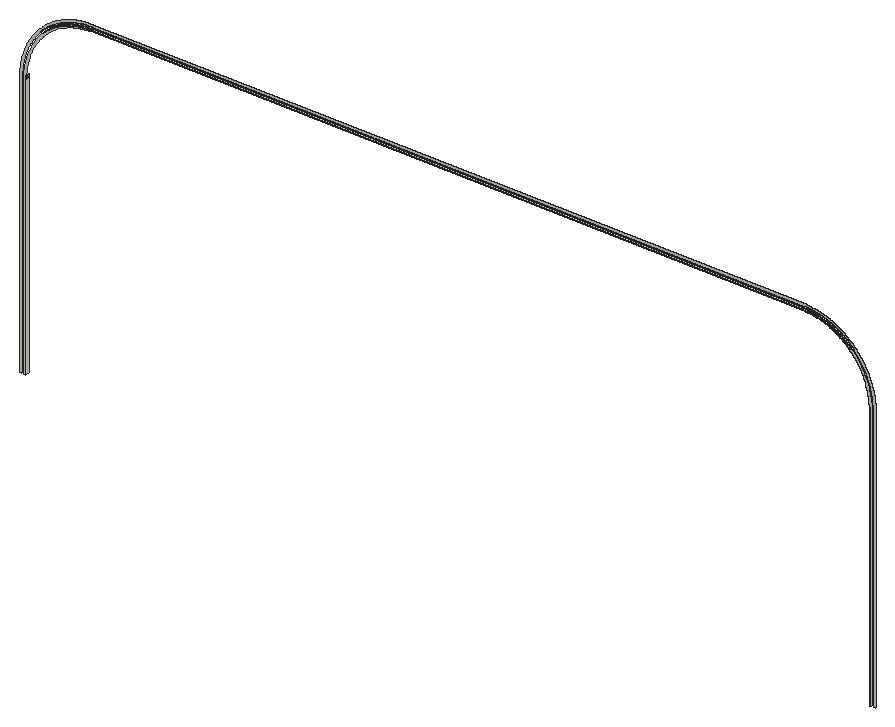
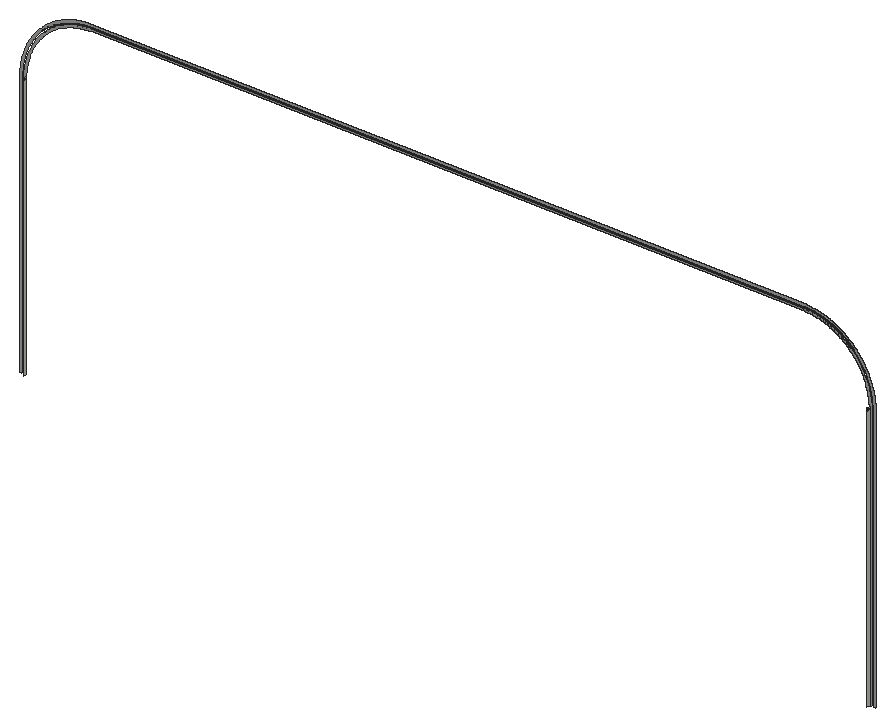
# SketchUp Ruby script. Lengths in inches.
U = 1.inch
M = Sketchup.active_model
def pt(a) = Geom::Point3d.new(a.map { |v| v * U })
def face(e, loops, mat)
  f = e.add_face(loops[0].map { |a| pt(a) })
  loops[1..].each { |l| e.add_face(l.map { |a| pt(a) }).erase! }
  f.material = f.back_material = mat if mat
  f
end
# faces: each face lists its corners as indices into pts; further lists are holes
def faces(e, pts, list, mat = nil) = list.each { |f| face(e, (f[0].is_a?(Array) ? f : [f]).map { |l| l.map { |i| pts[i] } }, mat) }
# xy, xz, yz: faces in a plane at the given z, y or x. An outline is a flat list of corners, or four numbers for a rectangle; further outlines are holes
def ring(l) = l.size == 4 ? [[l[0], l[1]], [l[2], l[1]], [l[2], l[3]], [l[0], l[3]]] : l.each_slice(2).to_a
def flat(e, list, mat, &to3) = list.each { |f| face(e, (f[0].is_a?(Array) ? f : [f]).map { |l| ring(l).map { |u, v| to3.(u, v) } }, mat) }
def xy(e, z, list, mat = nil) = flat(e, list, mat) { |x, y| [x, y, z] }
def xz(e, y, list, mat = nil) = flat(e, list, mat) { |x, z| [x, y, z] }
def yz(e, x, list, mat = nil) = flat(e, list, mat) { |y, z| [x, y, z] }
def lines(e, pts, list) = list.each { |a, b| e.add_line(pt(pts[a]), pt(pts[b])) }
# prism: a flat outline (further loops are holes) pulled along v
def prism(e, loops, v, mat = nil)
  f = face(e, loops, mat); d = Geom::Vector3d.new(v.map { |x| x * U })
  f.pushpull(f.normal.samedirection?(d) ? d.length : -d.length)
end
def box(e, o, s, mat = nil) = prism(e, [[o, [o[0] + s[0], o[1], o[2]], [o[0] + s[0], o[1] + s[1], o[2]], [o[0], o[1] + s[1], o[2]]]], [0, 0, s[2]], mat)
def at(x, y, z, deg = 0) = Geom::Transformation.translation(pt([x, y, z])) * Geom::Transformation.rotation(ORIGIN, Z_AXIS, deg.degrees)
def axes(o, x, y, z) = Geom::Transformation.new([*x, 0, *y, 0, *z, 0, *pt(o).to_a, 1])
def part(name) = M.definitions.add(name)
# library, detail: a bought-in or finely detailed component or shape, given as its bounding box
def library(name, o, s) = part(name).tap { |d| box(d.entities, o, s) }
def detail(e, o, s) = box(e.add_group.entities, o, s)
def put(e, d, t, mat = nil) = e.add_instance(d, t).tap { |i| i.material = mat if mat }
def group(e, t, mat = nil) = e.add_group.tap { |g| g.transformation = t; g.material = mat if mat }.entities
root = M.entities
M.materials.add("[Stone Vein Gray]").color = [206, 202, 201]
xy(root,52.84,[[183.43,83.25,183.57,83.5],[297.43,83.25,297.57,83.5]])
xy(root,52.85,[[183.72,83.25,183.86,83.5],[183.86,83.25,184,83.5],[184,83.25,297,83.5],[297,83.25,297.14,83.5],[297.14,83.25,297.28,83.5]])
xy(root,53.15,[[183.71,83.25,183.85,83.5],[183.85,83.25,184,83.5],[184,83.25,297,83.5],[297,83.25,297.15,83.5],[297.15,83.25,297.29,83.5]])
xz(root,83.5,[[172.5,0,172.5,42.3,172.52,42.6,172.52,42.75,172.54,42.9,172.55,43.05,172.5625,43.2,172.58,43.35,172.64,43.8,172.67,43.95,172.69,44.1,172.72,44.24,172.78,44.54,172.82,44.68,172.85,44.83,172.89,44.98,172.93,45.12,172.97,45.27,173.02,45.41,173.0625,45.55,173.11,45.7,173.26,46.12,173.32,46.26,173.43,46.54,173.49,46.68,173.56,46.81,173.62,46.95,173.6875,47.09,173.75,47.22,173.82,47.35,173.89,47.49,173.97,47.62,174.04,47.75,174.12,47.88,174.19,48.01,174.27,48.14,174.36,48.26,174.4375,48.39,174.52,48.51,174.61,48.64,174.79,48.88,174.875,49,174.97,49.12,175.0625,49.24,175.16,49.35,175.26,49.47,175.35,49.58,175.45,49.7,175.56,49.81,175.66,49.92,176.08,50.34,176.19,50.44,176.3,50.55,176.42,50.65,176.53,50.74,176.65,50.84,176.76,50.9375,176.88,51.03,177,51.125,177.12,51.21,177.36,51.39,177.49,51.48,177.61,51.5625,177.74,51.64,177.86,51.73,177.99,51.81,178.12,51.88,178.25,51.96,178.38,52.03,178.51,52.11,178.65,52.18,178.78,52.25,178.91,52.3125,179.05,52.38,179.19,52.44,179.32,52.51,179.46,52.57,179.74,52.68,179.88,52.74,180.3,52.89,180.45,52.9375,180.59,52.98,180.73,53.03,180.88,53.07,181.02,53.11,181.17,53.15,181.32,53.18,181.46,53.22,181.76,53.28,181.9,53.31,182.05,53.33,182.2,53.36,182.65,53.42,182.8,53.4375,182.95,53.45,183.1,53.46,183.25,53.48,183.4,53.48,183.7,53.5,297.3,53.5,297.6,53.48,297.75,53.48,297.9,53.46,298.05,53.45,298.2,53.4375,298.35,53.42,298.8,53.36,298.95,53.33,299.1,53.31,299.24,53.28,299.54,53.22,299.68,53.18,299.83,53.15,299.98,53.11,300.12,53.07,300.27,53.03,300.41,52.98,300.55,52.9375,300.7,52.89,301.12,52.74,301.26,52.68,301.54,52.57,301.68,52.51,301.81,52.44,301.95,52.38,302.09,52.3125,302.22,52.25,302.35,52.18,302.49,52.11,302.62,52.03,302.75,51.96,302.88,51.88,303.01,51.81,303.14,51.73,303.26,51.64,303.39,51.5625,303.51,51.48,303.64,51.39,303.88,51.21,304,51.125,304.12,51.03,304.24,50.9375,304.35,50.84,304.47,50.74,304.58,50.65,304.7,50.55,304.81,50.44,304.92,50.34,305.34,49.92,305.44,49.81,305.55,49.7,305.65,49.58,305.74,49.47,305.84,49.35,305.9375,49.24,306.03,49.12,306.125,49,306.21,48.88,306.39,48.64,306.48,48.51,306.5625,48.39,306.64,48.26,306.73,48.14,306.81,48.01,306.88,47.88,306.96,47.75,307.03,47.62,307.11,47.49,307.18,47.35,307.25,47.22,307.3125,47.09,307.38,46.95,307.44,46.81,307.51,46.68,307.57,46.54,307.68,46.26,307.74,46.12,307.89,45.7,307.9375,45.55,307.98,45.41,308.03,45.27,308.07,45.12,308.11,44.98,308.15,44.83,308.18,44.68,308.22,44.54,308.28,44.24,308.31,44.1,308.33,43.95,308.36,43.8,308.42,43.35,308.4375,43.2,308.45,43.05,308.46,42.9,308.48,42.75,308.48,42.6,308.5,42.3,308.5,0,308.15,0,308.15,42.29,308.14,42.4375,308.13,42.58,308.125,42.73,308.12,42.875,308.1,43.02,308.09,43.17,308.07,43.3125,308.05,43.46,308.01,43.74,307.99,43.89,307.96,44.03,307.9375,44.18,307.91,44.32,307.84,44.6,307.81,44.74,307.77,44.89,307.65,45.31,307.6,45.45,307.56,45.58,307.41,46,307.36,46.13,307.3,46.27,307.24,46.4,307.1875,46.54,307,46.93,306.93,47.0625,306.87,47.19,306.66,47.58,306.58,47.7,306.51,47.83,306.27,48.19,306.1875,48.32,306.11,48.44,306.02,48.55,305.93,48.67,305.85,48.79,305.76,48.9,305.67,49.02,305.57,49.13,305.48,49.24,305.38,49.35,305.29,49.46,305.1875,49.57,305.09,49.68,304.99,49.78,304.88,49.88,304.78,49.99,304.68,50.09,304.57,50.1875,304.46,50.29,304.35,50.38,304.24,50.48,304.13,50.57,304.02,50.67,303.9,50.76,303.79,50.85,303.67,50.93,303.55,51.02,303.44,51.11,303.32,51.1875,303.19,51.27,302.83,51.51,302.7,51.58,302.58,51.66,302.19,51.87,302.0625,51.93,301.93,52,301.54,52.1875,301.4,52.24,301.27,52.3,301.13,52.36,301,52.41,300.58,52.56,300.45,52.6,300.31,52.65,299.89,52.77,299.74,52.81,299.6,52.84,299.32,52.91,299.18,52.9375,299.03,52.96,298.89,52.99,298.74,53.01,298.46,53.05,298.3125,53.07,298.17,53.09,298.02,53.1,297.875,53.12,297.73,53.125,297.58,53.13,297.4375,53.14,297.29,53.15,183.71,53.15,183.5625,53.14,183.42,53.13,183.27,53.125,183.125,53.12,182.98,53.1,182.83,53.09,182.6875,53.07,182.54,53.05,182.26,53.01,182.11,52.99,181.97,52.96,181.82,52.9375,181.68,52.91,181.4,52.84,181.26,52.81,181.11,52.77,180.69,52.65,180.55,52.6,180.42,52.56,180,52.41,179.87,52.36,179.73,52.3,179.6,52.24,179.46,52.1875,179.07,52,178.9375,51.93,178.81,51.87,178.42,51.66,178.3,51.58,178.17,51.51,177.81,51.27,177.68,51.1875,177.56,51.11,177.45,51.02,177.33,50.93,177.21,50.85,177.1,50.76,176.98,50.67,176.87,50.57,176.76,50.48,176.65,50.38,176.54,50.29,176.43,50.1875,176.32,50.09,176.22,49.99,176.12,49.88,176.01,49.78,175.91,49.68,175.8125,49.57,175.71,49.46,175.62,49.35,175.52,49.24,175.43,49.13,175.33,49.02,175.24,48.9,175.15,48.79,175.07,48.67,174.98,48.55,174.89,48.44,174.8125,48.32,174.73,48.19,174.49,47.83,174.42,47.7,174.34,47.57,174.27,47.45,174.13,47.19,174.07,47.0625,174,46.93,173.8125,46.54,173.76,46.4,173.7,46.27,173.64,46.13,173.59,46,173.44,45.58,173.4,45.45,173.35,45.31,173.23,44.89,173.19,44.74,173.16,44.6,173.09,44.32,173.0625,44.18,173.04,44.03,173.01,43.89,172.99,43.74,172.95,43.46,172.93,43.3125,172.91,43.17,172.9,43.02,172.88,42.875,172.875,42.73,172.87,42.58,172.86,42.4375,172.85,42.29,172.85,0],[173.15,0,173.15,42.28,173.16,42.43,173.16,42.57,173.18,42.85,173.2,42.99,173.21,43.13,173.23,43.28,173.24,43.42,173.28,43.7,173.31,43.84,173.33,43.98,173.39,44.26,173.42,44.39,173.48,44.67,173.56,44.95,173.6,45.08,173.64,45.22,173.68,45.35,173.73,45.49,173.77,45.62,173.82,45.76,173.92,46.02,173.98,46.15,174.03,46.28,174.33,46.93,174.4,47.05,174.46,47.18,174.6,47.42,174.68,47.55,174.82,47.79,175.06,48.15,175.14,48.26,175.22,48.38,175.31,48.49,175.39,48.61,175.57,48.83,175.66,48.9375,175.75,49.05,175.84,49.15,175.9375,49.26,176.03,49.36,176.13,49.47,176.53,49.87,176.64,49.97,176.74,50.0625,176.85,50.16,176.95,50.25,177.0625,50.34,177.17,50.43,177.39,50.61,177.51,50.69,177.62,50.78,177.74,50.86,177.85,50.94,178.21,51.18,178.45,51.32,178.58,51.4,178.82,51.54,178.95,51.6,179.07,51.67,179.72,51.97,179.85,52.02,179.98,52.08,180.24,52.18,180.38,52.23,180.51,52.27,180.65,52.32,180.78,52.36,180.92,52.4,181.05,52.44,181.33,52.52,181.61,52.58,181.74,52.61,182.02,52.67,182.16,52.69,182.3,52.72,182.58,52.76,182.72,52.77,182.87,52.79,183.01,52.8,183.15,52.82,183.43,52.84,183.57,52.84,183.72,52.85,297.28,52.85,297.43,52.84,297.57,52.84,297.85,52.82,297.99,52.8,298.13,52.79,298.28,52.77,298.42,52.76,298.7,52.72,298.84,52.69,298.98,52.67,299.26,52.61,299.39,52.58,299.67,52.52,299.95,52.44,300.08,52.4,300.22,52.36,300.35,52.32,300.49,52.27,300.62,52.23,300.76,52.18,301.02,52.08,301.15,52.02,301.28,51.97,301.93,51.67,302.05,51.6,302.18,51.54,302.42,51.4,302.55,51.32,302.79,51.18,303.15,50.94,303.26,50.86,303.38,50.78,303.49,50.69,303.61,50.61,303.83,50.43,303.9375,50.34,304.05,50.25,304.15,50.16,304.26,50.0625,304.36,49.97,304.47,49.87,304.87,49.47,304.97,49.36,305.0625,49.26,305.16,49.15,305.25,49.05,305.34,48.9375,305.43,48.83,305.61,48.61,305.69,48.49,305.78,48.38,305.86,48.26,305.94,48.15,306.18,47.79,306.32,47.55,306.4,47.43,306.47,47.3,306.54,47.18,306.6,47.05,306.67,46.93,306.97,46.28,307.02,46.15,307.08,46.02,307.18,45.76,307.23,45.62,307.27,45.49,307.32,45.35,307.36,45.22,307.4,45.08,307.44,44.95,307.52,44.67,307.58,44.39,307.61,44.26,307.67,43.98,307.69,43.84,307.72,43.7,307.76,43.42,307.77,43.28,307.79,43.13,307.8,42.99,307.82,42.85,307.84,42.57,307.84,42.43,307.85,42.28,307.85,0,307.5,0,307.5,42.27,307.49,42.41,307.49,42.55,307.48,42.6875,307.47,42.82,307.46,42.96,307.44,43.1,307.43,43.23,307.39,43.51,307.37,43.64,307.35,43.78,307.32,43.91,307.3,44.05,307.27,44.18,307.24,44.32,307.18,44.58,307.14,44.72,307.11,44.85,306.99,45.24,306.94,45.375,306.9,45.5,306.7,46.02,306.65,46.14,306.59,46.27,306.54,46.4,306.42,46.64,306.36,46.77,306.29,46.89,306.23,47.01,305.95,47.49,305.88,47.6,305.81,47.72,305.73,47.83,305.65,47.95,305.25,48.5,305.16,48.61,305.07,48.71,304.98,48.82,304.89,48.92,304.8,49.03,304.62,49.23,304.52,49.33,304.42,49.42,304.33,49.52,304.23,49.62,304.03,49.8,303.92,49.89,303.82,49.98,303.71,50.07,303.61,50.16,303.5,50.25,302.95,50.65,302.83,50.73,302.72,50.81,302.6,50.88,302.49,50.95,302.01,51.23,301.89,51.29,301.77,51.36,301.64,51.42,301.4,51.54,301.27,51.59,301.14,51.65,301.02,51.7,300.5,51.9,300.375,51.94,300.24,51.99,299.85,52.11,299.72,52.14,299.58,52.18,299.32,52.24,299.18,52.27,299.05,52.3,298.91,52.32,298.78,52.35,298.64,52.37,298.51,52.39,298.23,52.43,298.1,52.44,297.96,52.46,297.82,52.47,297.6875,52.48,297.55,52.49,297.41,52.49,297.27,52.5,183.73,52.5,183.59,52.49,183.45,52.49,183.3125,52.48,183.18,52.47,183.04,52.46,182.9,52.44,182.77,52.43,182.49,52.39,182.36,52.37,182.22,52.35,182.09,52.32,181.95,52.3,181.82,52.27,181.68,52.24,181.42,52.18,181.28,52.14,181.15,52.11,180.76,51.99,180.625,51.94,180.5,51.9,179.98,51.7,179.86,51.65,179.73,51.59,179.6,51.54,179.36,51.42,179.23,51.36,179.11,51.29,178.99,51.23,178.51,50.95,178.4,50.88,178.28,50.81,178.17,50.73,178.05,50.65,177.5,50.25,177.39,50.16,177.29,50.07,177.18,49.98,177.08,49.89,176.97,49.8,176.77,49.62,176.67,49.52,176.58,49.42,176.48,49.33,176.38,49.23,176.2,49.03,176.11,48.92,176.02,48.82,175.93,48.71,175.84,48.61,175.75,48.5,175.35,47.95,175.27,47.83,175.19,47.72,175.12,47.6,175.05,47.49,174.77,47.01,174.71,46.89,174.64,46.77,174.58,46.64,174.46,46.4,174.41,46.27,174.35,46.14,174.3,46.02,174.1,45.5,174.06,45.375,174.01,45.24,173.89,44.85,173.86,44.72,173.82,44.58,173.76,44.32,173.73,44.18,173.7,44.05,173.68,43.91,173.65,43.78,173.63,43.64,173.61,43.51,173.57,43.23,173.56,43.1,173.54,42.96,173.53,42.82,173.52,42.6875,173.51,42.55,173.51,42.41,173.5,42.27,173.5,0]],"[Stone Vein Gray]")
yz(root,173.5,[[83.5,0,84,42],[83.5,42,84,42.14],[83.5,42.14,84,42.27]])
yz(root,173.51,[[83.5,42.41,84,42.55]])
yz(root,307.5,[[83.5,0,84,42],[83.5,42,84,42.14],[83.5,42.14,84,42.27]])
p = [[173.51,84,42.41],[173.5,84,42.27],[173.5,83.5,42.27],[173.51,83.5,42.41],[307.5,84,42.27],[307.49,84,42.41],
  [307.49,83.5,42.41],[307.5,83.5,42.27],[176.01,83.5,49.78],[176.12,83.5,49.88],[176.12,83.25,49.88],[176.01,83.25,49.78],
  [304.57,83.5,49.77],[304.47,83.5,49.87],[304.47,83.25,49.87],[304.57,83.25,49.77],[304.88,83.5,49.88],[304.99,83.5,49.78],
  [304.99,83.25,49.78],[304.88,83.25,49.88],[176.22,83.5,49.99],[176.22,83.25,49.99],[176.64,83.5,49.97],[176.53,83.5,49.87],
  [176.53,83.25,49.87],[176.64,83.25,49.97],[304.36,83.5,49.97],[304.36,83.25,49.97],[304.78,83.5,49.99],[304.78,83.25,49.99],
  [176.32,83.5,50.09],[176.32,83.25,50.09],[176.74,83.5,50.0625],[176.74,83.25,50.0625],[304.26,83.5,50.0625],[304.26,83.25,50.0625],
  [304.68,83.5,50.09],[304.68,83.25,50.09],[176.43,83.5,50.1875],[176.43,83.25,50.1875],[176.85,83.5,50.16],[176.85,83.25,50.16],
  [304.15,83.5,50.16],[304.15,83.25,50.16],[304.57,83.5,50.1875],[304.57,83.25,50.1875],[176.54,83.5,50.29],[176.54,83.25,50.29],
  [176.95,83.5,50.25],[176.95,83.25,50.25],[304.05,83.5,50.25],[304.05,83.25,50.25],[304.46,83.5,50.29],[304.46,83.25,50.29],
  [176.65,83.5,50.38],[176.65,83.25,50.38],[177.0625,83.5,50.34],[177.0625,83.25,50.34],[177.17,83.5,50.43],[177.17,83.25,50.43],
  [303.9375,83.5,50.34],[303.83,83.5,50.43],[303.83,83.25,50.43],[303.9375,83.25,50.34],[304.35,83.5,50.38],[304.35,83.25,50.38],
  [176.76,83.5,50.48],[176.76,83.25,50.48],[177.28,83.5,50.52],[177.28,83.25,50.52],[303.72,83.5,50.52],[303.72,83.25,50.52],
  [304.24,83.5,50.48],[304.24,83.25,50.48],[176.87,83.5,50.57],[176.87,83.25,50.57],[177.39,83.5,50.61],[177.39,83.25,50.61],
  [303.61,83.5,50.61],[303.61,83.25,50.61],[304.13,83.5,50.57],[304.13,83.25,50.57],[176.98,83.5,50.67],[176.98,83.25,50.67],
  [177.51,83.5,50.69],[177.51,83.25,50.69],[303.49,83.5,50.69],[303.49,83.25,50.69],[304.02,83.5,50.67],[304.02,83.25,50.67],
  [177.1,83.5,50.76],[177.1,83.25,50.76],[177.62,83.5,50.78],[177.62,83.25,50.78],[303.38,83.5,50.78],[303.38,83.25,50.78],
  [303.9,83.5,50.76],[303.9,83.25,50.76],[177.21,83.5,50.85],[177.21,83.25,50.85],[177.33,83.5,50.93],[177.33,83.25,50.93],
  [177.74,83.5,50.86],[177.74,83.25,50.86],[303.26,83.5,50.86],[303.26,83.25,50.86],[303.67,83.5,50.93],[303.79,83.5,50.85],
  [303.79,83.25,50.85],[303.67,83.25,50.93],[177.45,83.5,51.02],[177.45,83.25,51.02],[177.85,83.5,50.94],[177.85,83.25,50.94],
  [177.97,83.5,51.02],[177.97,83.25,51.02],[303.15,83.5,50.94],[303.03,83.5,51.02],[303.03,83.25,51.02],[303.15,83.25,50.94],
  [303.55,83.5,51.02],[303.55,83.25,51.02],[177.56,83.5,51.11],[177.56,83.25,51.11],[178.09,83.5,51.1],[178.09,83.25,51.1],
  [302.91,83.5,51.1],[302.91,83.25,51.1],[303.44,83.5,51.11],[303.44,83.25,51.11],[177.68,83.5,51.1875],[177.68,83.25,51.1875],
  [178.21,83.5,51.18],[178.21,83.25,51.18],[302.79,83.5,51.18],[302.79,83.25,51.18],[303.32,83.5,51.1875],[303.32,83.25,51.1875],
  [177.81,83.5,51.27],[177.81,83.25,51.27],[178.33,83.5,51.25],[178.33,83.25,51.25],[302.67,83.5,51.25],[302.67,83.25,51.25],
  [303.19,83.5,51.27],[303.19,83.25,51.27],[177.93,83.5,51.35],[177.93,83.25,51.35],[178.45,83.5,51.32],[178.45,83.25,51.32],
  [178.58,83.5,51.4],[178.58,83.25,51.4],[302.55,83.5,51.32],[302.42,83.5,51.4],[302.42,83.25,51.4],[302.55,83.25,51.32],
  [303.07,83.5,51.35],[303.07,83.25,51.35],[178.05,83.5,51.43],[178.05,83.25,51.43],[178.17,83.5,51.51],[178.17,83.25,51.51],
  [178.7,83.5,51.47],[178.7,83.25,51.47],[302.3,83.5,51.47],[302.3,83.25,51.47],[302.83,83.5,51.51],[302.95,83.5,51.43],
  [302.95,83.25,51.43],[302.83,83.25,51.51],[178.3,83.5,51.58],[178.3,83.25,51.58],[178.82,83.5,51.54],[178.82,83.25,51.54],
  [178.95,83.5,51.6],[178.95,83.25,51.6],[302.18,83.5,51.54],[302.05,83.5,51.6],[302.05,83.25,51.6],[302.18,83.25,51.54],
  [302.7,83.5,51.58],[302.7,83.25,51.58],[178.42,83.5,51.66],[178.42,83.25,51.66],[179.07,83.5,51.67],[179.07,83.25,51.67],
  [301.93,83.5,51.67],[301.93,83.25,51.67],[302.58,83.5,51.66],[302.58,83.25,51.66],[178.55,83.5,51.73],[178.55,83.25,51.73],
  [178.68,83.5,51.8],[178.68,83.25,51.8],[179.2,83.5,51.73],[179.2,83.25,51.73],[179.33,83.5,51.79],[179.33,83.25,51.79],
  [301.8,83.5,51.73],[301.67,83.5,51.79],[301.67,83.25,51.79],[301.8,83.25,51.73],[302.32,83.5,51.8],[302.45,83.5,51.73],
  [302.45,83.25,51.73],[302.32,83.25,51.8],[178.81,83.5,51.87],[178.81,83.25,51.87],[179.46,83.5,51.85],[179.46,83.25,51.85],
  [301.54,83.5,51.85],[301.54,83.25,51.85],[302.19,83.5,51.87],[302.19,83.25,51.87],[178.9375,83.5,51.93],[178.9375,83.25,51.93],
  [179.07,83.5,52],[179.07,83.25,52],[179.59,83.5,51.91],[179.59,83.25,51.91],[179.72,83.5,51.97],[179.72,83.25,51.97],
  [301.41,83.5,51.91],[301.28,83.5,51.97],[301.28,83.25,51.97],[301.41,83.25,51.91],[301.93,83.5,52],[302.0625,83.5,51.93],
  [302.0625,83.25,51.93],[301.93,83.25,52],[179.2,83.5,52.0625],[179.2,83.25,52.0625],[179.85,83.5,52.02],[179.85,83.25,52.02],
  [179.98,83.5,52.08],[179.98,83.25,52.08],[301.15,83.5,52.02],[301.02,83.5,52.08],[301.02,83.25,52.08],[301.15,83.25,52.02],
  [301.8,83.5,52.0625],[301.8,83.25,52.0625],[179.33,83.5,52.125],[179.33,83.25,52.125],[179.46,83.5,52.1875],[179.46,83.25,52.1875],
  [180.11,83.5,52.13],[180.11,83.25,52.13],[180.24,83.5,52.18],[180.24,83.25,52.18],[300.89,83.5,52.13],[300.76,83.5,52.18],
  [300.76,83.25,52.18],[300.89,83.25,52.13],[301.54,83.5,52.1875],[301.67,83.5,52.125],[301.67,83.25,52.125],[301.54,83.25,52.1875],
  [179.6,83.5,52.24],[179.6,83.25,52.24],[179.73,83.5,52.3],[179.73,83.25,52.3],[180.38,83.5,52.23],[180.38,83.25,52.23],
  [180.51,83.5,52.27],[180.51,83.25,52.27],[300.62,83.5,52.23],[300.49,83.5,52.27],[300.49,83.25,52.27],[300.62,83.25,52.23],
  [301.27,83.5,52.3],[301.4,83.5,52.24],[301.4,83.25,52.24],[301.27,83.25,52.3],[179.87,83.5,52.36],[179.87,83.25,52.36],
  [180.65,83.5,52.32],[180.65,83.25,52.32],[180.78,83.5,52.36],[180.78,83.25,52.36],[300.35,83.5,52.32],[300.22,83.5,52.36],
  [300.22,83.25,52.36],[300.35,83.25,52.32],[301.13,83.5,52.36],[301.13,83.25,52.36],[180,83.5,52.41],[180,83.25,52.41],
  [180.14,83.5,52.46],[180.14,83.25,52.46],[180.92,83.5,52.4],[180.92,83.25,52.4],[181.05,83.5,52.44],[181.05,83.25,52.44],
  [181.19,83.5,52.48],[181.19,83.25,52.48],[299.95,83.5,52.44],[299.81,83.5,52.48],[299.81,83.25,52.48],[299.95,83.25,52.44],
  [300.08,83.5,52.4],[300.08,83.25,52.4],[300.86,83.5,52.46],[301,83.5,52.41],[301,83.25,52.41],[300.86,83.25,52.46],
  [180.28,83.5,52.51],[180.28,83.25,52.51],[180.42,83.5,52.56],[180.42,83.25,52.56],[181.33,83.5,52.52],[181.33,83.25,52.52],
  [181.47,83.5,52.55],[181.47,83.25,52.55],[299.67,83.5,52.52],[299.53,83.5,52.55],[299.53,83.25,52.55],[299.67,83.25,52.52],
  [300.58,83.5,52.56],[300.72,83.5,52.51],[300.72,83.25,52.51],[300.58,83.25,52.56],[180.55,83.5,52.6],[180.55,83.25,52.6],
  [180.69,83.5,52.65],[180.69,83.25,52.65],[180.83,83.5,52.69],[180.83,83.25,52.69],[181.61,83.5,52.58],[181.61,83.25,52.58],
  [181.74,83.5,52.61],[181.74,83.25,52.61],[181.88,83.5,52.64],[181.88,83.25,52.64],[182.02,83.5,52.67],[182.02,83.25,52.67],
  [299.12,83.5,52.64],[298.98,83.5,52.67],[298.98,83.25,52.67],[299.12,83.25,52.64],[299.26,83.5,52.61],[299.26,83.25,52.61],
  [299.39,83.5,52.58],[299.39,83.25,52.58],[300.17,83.5,52.69],[300.31,83.5,52.65],[300.31,83.25,52.65],[300.17,83.25,52.69],
  [300.45,83.5,52.6],[300.45,83.25,52.6],[180.97,83.5,52.73],[180.97,83.25,52.73],[181.11,83.5,52.77],[181.11,83.25,52.77],
  [182.16,83.5,52.69],[182.16,83.25,52.69],[182.3,83.5,52.72],[182.3,83.25,52.72],[182.44,83.5,52.74],[182.44,83.25,52.74],
  [182.58,83.5,52.76],[182.58,83.25,52.76],[298.56,83.5,52.74],[298.42,83.5,52.76],[298.42,83.25,52.76],[298.56,83.25,52.74],
  [298.7,83.5,52.72],[298.7,83.25,52.72],[298.84,83.5,52.69],[298.84,83.25,52.69],[299.89,83.5,52.77],[300.03,83.5,52.73],
  [300.03,83.25,52.73],[299.89,83.25,52.77],[181.26,83.5,52.81],[181.26,83.25,52.81],[181.4,83.5,52.84],[181.4,83.25,52.84],
  [181.54,83.5,52.875],[181.54,83.25,52.875],[182.72,83.5,52.77],[182.72,83.25,52.77],[182.87,83.5,52.79],[182.87,83.25,52.79],
  [183.01,83.5,52.8],[183.01,83.25,52.8],[183.15,83.5,52.82],[183.15,83.25,52.82],[183.29,83.5,52.83],[183.29,83.25,52.83],
  [183.43,83.5,52.84],[183.43,83.25,52.84],[183.72,83.5,52.85],[183.57,83.5,52.84],[183.57,83.25,52.84],[183.72,83.25,52.85],
  [297.43,83.5,52.84],[297.28,83.5,52.85],[297.28,83.25,52.85],[297.43,83.25,52.84],[297.71,83.5,52.83],[297.57,83.5,52.84],
  [297.57,83.25,52.84],[297.71,83.25,52.83],[297.85,83.5,52.82],[297.85,83.25,52.82],[297.99,83.5,52.8],[297.99,83.25,52.8],
  [298.13,83.5,52.79],[298.13,83.25,52.79],[298.28,83.5,52.77],[298.28,83.25,52.77],[299.46,83.5,52.875],[299.6,83.5,52.84],
  [299.6,83.25,52.84],[299.46,83.25,52.875],[299.74,83.5,52.81],[299.74,83.25,52.81],[181.68,83.5,52.91],[181.68,83.25,52.91],
  [181.82,83.5,52.9375],[181.82,83.25,52.9375],[181.97,83.5,52.96],[181.97,83.25,52.96],[299.03,83.5,52.96],[299.18,83.5,52.9375],
  [299.18,83.25,52.9375],[299.03,83.25,52.96],[299.32,83.5,52.91],[299.32,83.25,52.91],[182.11,83.5,52.99],[182.11,83.25,52.99],
  [182.26,83.5,53.01],[182.26,83.25,53.01],[182.4,83.5,53.03],[182.4,83.25,53.03],[182.54,83.5,53.05],[182.54,83.25,53.05],
  [298.46,83.5,53.05],[298.6,83.5,53.03],[298.6,83.25,53.03],[298.46,83.25,53.05],[298.74,83.5,53.01],[298.74,83.25,53.01],
  [298.89,83.5,52.99],[298.89,83.25,52.99],[182.6875,83.5,53.07],[182.6875,83.25,53.07],[182.83,83.5,53.09],[182.83,83.25,53.09],
  [182.98,83.5,53.1],[182.98,83.25,53.1],[183.125,83.5,53.12],[183.125,83.25,53.12],[183.27,83.5,53.125],[183.27,83.25,53.125],
  [183.42,83.5,53.13],[183.42,83.25,53.13],[183.5625,83.5,53.14],[183.5625,83.25,53.14],[183.71,83.5,53.15],[183.71,83.25,53.15],
  [297.29,83.5,53.15],[297.4375,83.5,53.14],[297.4375,83.25,53.14],[297.29,83.25,53.15],[297.58,83.5,53.13],[297.58,83.25,53.13],
  [297.73,83.5,53.125],[297.73,83.25,53.125],[297.875,83.5,53.12],[297.875,83.25,53.12],[298.02,83.5,53.1],[298.02,83.25,53.1],
  [298.17,83.5,53.09],[298.17,83.25,53.09],[298.3125,83.5,53.07],[298.3125,83.25,53.07]]
faces(root,p,[[0,1,2,3],[4,5,6,7],[8,9,10,11],[12,13,14,15],[16,17,18,19],[9,20,21,10],[22,23,24,25],[13,26,27,14],
  [28,16,19,29],[20,30,31,21],[32,22,25,33],[26,34,35,27],[36,28,29,37],[30,38,39,31],[40,32,33,41],[34,42,43,35],
  [44,36,37,45],[38,46,47,39],[48,40,41,49],[42,50,51,43],[52,44,45,53],[46,54,55,47],[56,48,49,57],[58,56,57,59],
  [60,61,62,63],[50,60,63,51],[64,52,53,65],[54,66,67,55],[68,58,59,69],[61,70,71,62],[72,64,65,73],[66,74,75,67],
  [76,68,69,77],[70,78,79,71],[80,72,73,81],[74,82,83,75],[84,76,77,85],[78,86,87,79],[88,80,81,89],[82,90,91,83],
  [92,84,85,93],[86,94,95,87],[96,88,89,97],[90,98,99,91],[98,100,101,99],[102,92,93,103],[94,104,105,95],[106,107,108,109],
  [107,96,97,108],[100,110,111,101],[112,102,103,113],[114,112,113,115],[116,117,118,119],[104,116,119,105],[120,106,109,121],[110,122,123,111],
  [124,114,115,125],[117,126,127,118],[128,120,121,129],[122,130,131,123],[132,124,125,133],[126,134,135,127],[136,128,129,137],[130,138,139,131],
  [140,132,133,141],[134,142,143,135],[144,136,137,145],[138,146,147,139],[148,140,141,149],[150,148,149,151],[152,153,154,155],[142,152,155,143],
  [156,144,145,157],[146,158,159,147],[158,160,161,159],[162,150,151,163],[153,164,165,154],[166,167,168,169],[167,156,157,168],[160,170,171,161],
  [172,162,163,173],[174,172,173,175],[176,177,178,179],[164,176,179,165],[180,166,169,181],[170,182,183,171],[184,174,175,185],[177,186,187,178],
  [188,180,181,189],[182,190,191,183],[190,192,193,191],[194,184,185,195],[196,194,195,197],[198,199,200,201],[186,198,201,187],[202,203,204,205],
  [203,188,189,204],[192,206,207,193],[208,196,197,209],[199,210,211,200],[212,202,205,213],[206,214,215,207],[214,216,217,215],[218,208,209,219],
  [220,218,219,221],[222,223,224,225],[210,222,225,211],[226,227,228,229],[227,212,213,228],[216,230,231,217],[232,220,221,233],[234,232,233,235],
  [236,237,238,239],[223,236,239,224],[240,226,229,241],[230,242,243,231],[242,244,245,243],[246,234,235,247],[248,246,247,249],[250,251,252,253],
  [237,250,253,238],[254,255,256,257],[255,240,241,256],[244,258,259,245],[258,260,261,259],[262,248,249,263],[264,262,263,265],[266,267,268,269],
  [251,266,269,252],[270,271,272,273],[271,254,257,272],[260,274,275,261],[276,264,265,277],[278,276,277,279],[280,281,282,283],[267,280,283,268],
  [284,270,273,285],[274,286,287,275],[286,288,289,287],[290,278,279,291],[292,290,291,293],[294,292,293,295],[296,297,298,299],[300,296,299,301],
  [281,300,301,282],[302,303,304,305],[303,284,285,304],[288,306,307,289],[306,308,309,307],[310,294,295,311],[312,310,311,313],[314,315,316,317],
  [297,314,317,298],[318,319,320,321],[319,302,305,320],[308,322,323,309],[322,324,325,323],[324,326,327,325],[328,312,313,329],[330,328,329,331],
  [332,330,331,333],[334,332,333,335],[336,337,338,339],[340,336,339,341],[342,340,341,343],[315,342,343,316],[344,345,346,347],[345,348,349,346],
  [348,318,321,349],[326,350,351,327],[350,352,353,351],[354,334,335,355],[356,354,355,357],[358,356,357,359],[360,358,359,361],[362,363,364,365],
  [366,362,365,367],[368,366,367,369],[337,368,369,338],[370,371,372,373],[371,344,347,372],[352,374,375,353],[374,376,377,375],[376,378,379,377],
  [380,360,361,381],[382,380,381,383],[384,382,383,385],[386,384,385,387],[388,386,387,389],[390,388,389,391],[392,393,394,395],[396,397,398,399],
  [400,401,402,403],[404,400,403,405],[406,404,405,407],[408,406,407,409],[410,408,409,411],[363,410,411,364],[412,413,414,415],[413,416,417,414],
  [416,370,373,417],[378,418,419,379],[418,420,421,419],[420,422,423,421],[424,425,426,427],[425,428,429,426],[428,412,415,429],[422,430,431,423],
  [430,432,433,431],[432,434,435,433],[434,436,437,435],[438,439,440,441],[439,442,443,440],[442,444,445,443],[444,424,427,445],[436,446,447,437],
  [446,448,449,447],[448,450,451,449],[450,452,453,451],[452,454,455,453],[454,456,457,455],[456,458,459,457],[458,460,461,459],[462,463,464,465],
  [463,466,467,464],[466,468,469,467],[468,470,471,469],[470,472,473,471],[472,474,475,473],[474,476,477,475],[476,438,441,477]])
